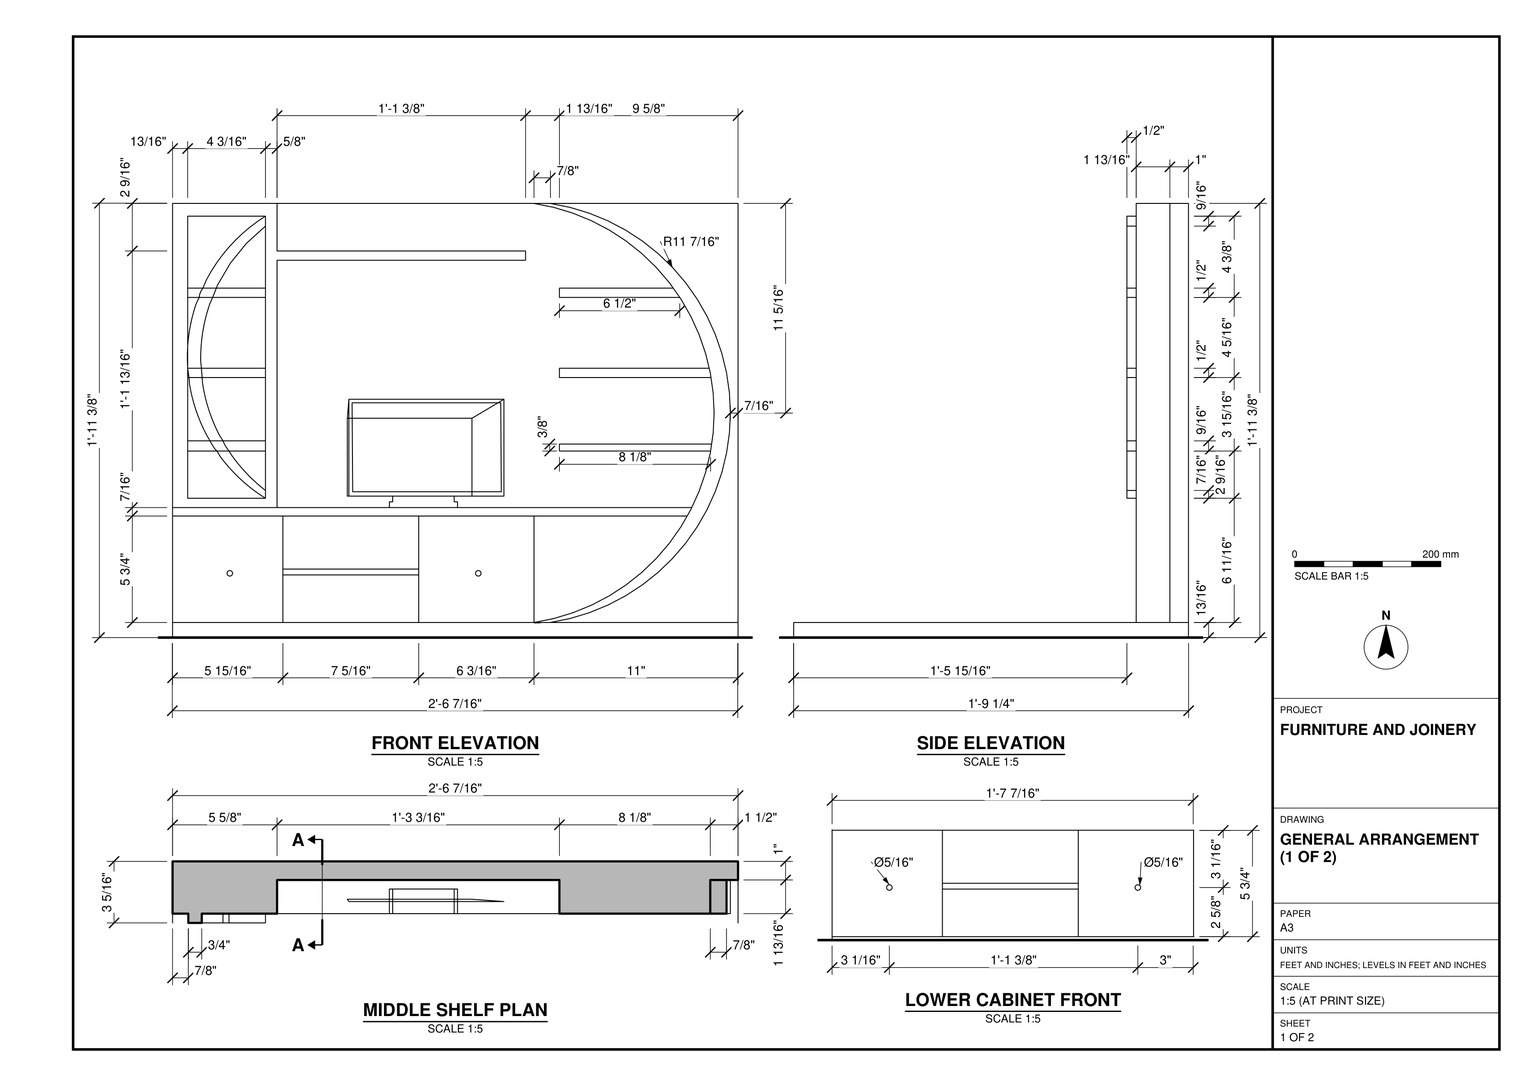
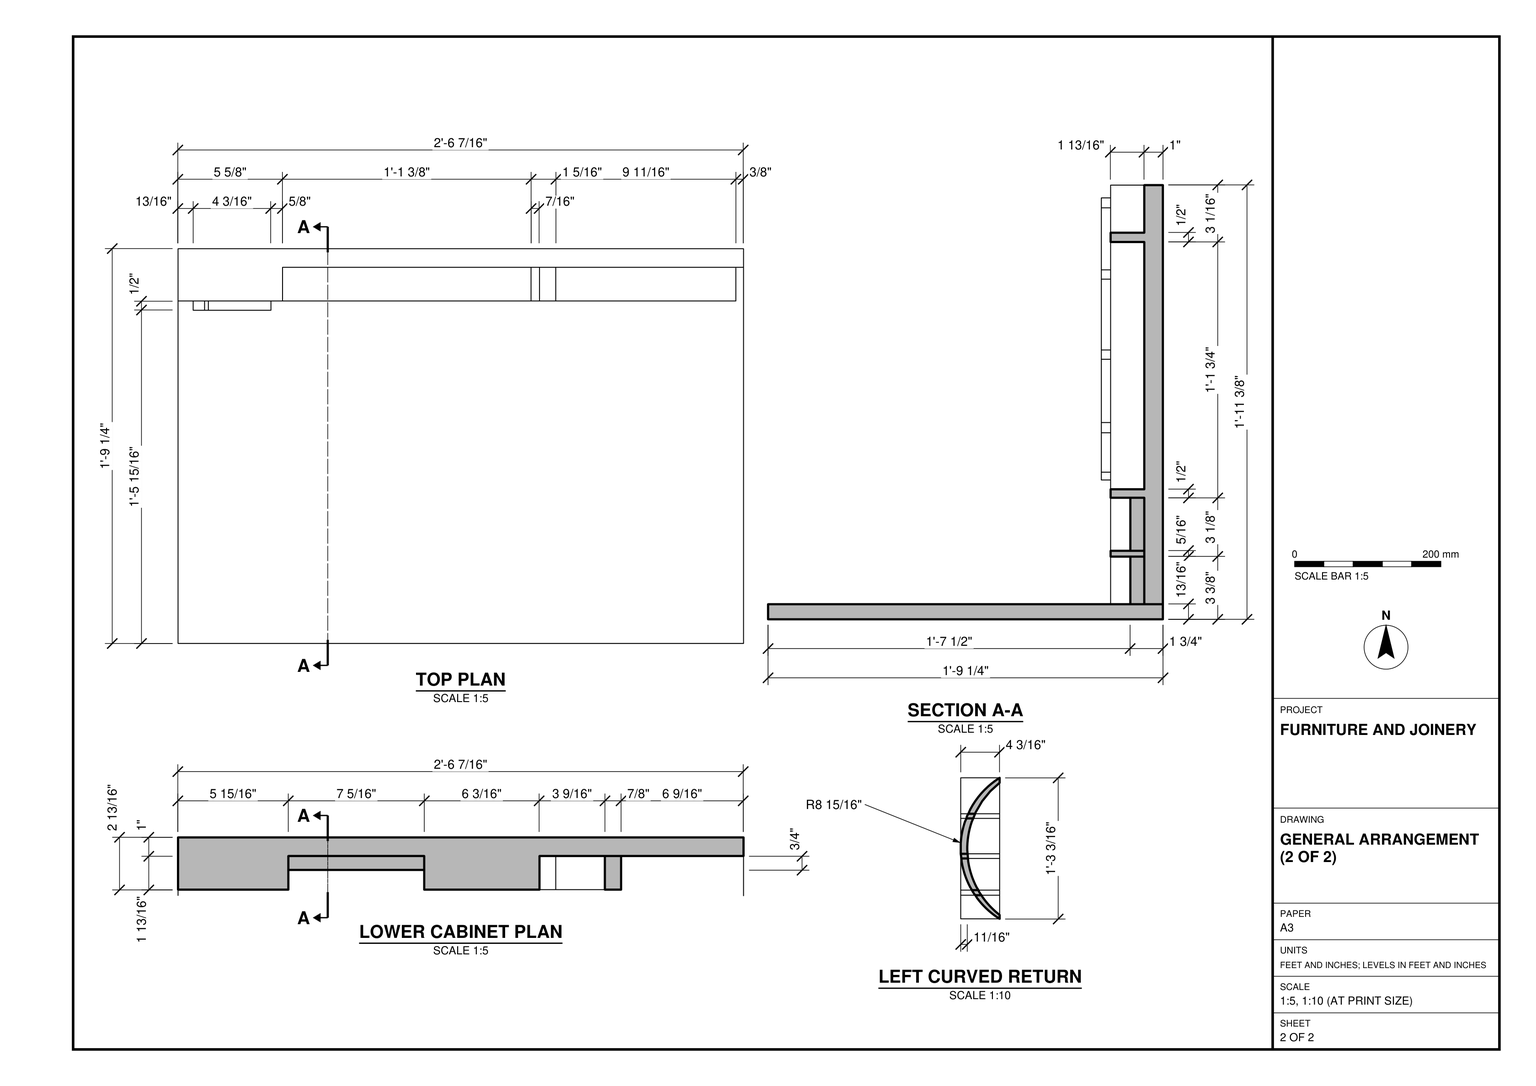
Use both sheets of task_files/diagram_01.pdf to model the television display unit in SketchUp. Work in feet and inches. Set the underside of the platform at ±0'-0". The complete unit is 2'-6 7/16" wide, 1'-9 1/4" deep and 1'-11 3/8" high. The depth includes the platform projecting in front of the shallow joinery; use the top plan and section to distinguish the platform footprint from the cabinet footprint.

Build the full-width platform and upright back panel. At the foot of the panel, place the lower cabinet with a knobbed front on either side of a recessed, shelved bay. Extend the display shelf above the cabinet to meet the large right-hand curve. Place the television on its stand in the central display space, with the short upper shelf extending into that space from the left. Use the curved-return detail for the narrow left shelving bay. On the right, follow the larger arc from the top of the unit down to the platform, fitting the three shelves to its inner edge.

Keep the platform, back panel, cabinet and other distinct joinery pieces in separate groups or components, and use components for repeated parts. Decor and loose items, including the television, may use any suitable library component. Save one SketchUp model as output_files/television_display_unit_with_curved_shelving.skp.

# SketchUp Ruby script. Lengths in inches.
U = 1.inch
M = Sketchup.active_model
def pt(a) = Geom::Point3d.new(a.map { |v| v * U })
def face(e, loops, mat)
  f = e.add_face(loops[0].map { |a| pt(a) })
  loops[1..].each { |l| e.add_face(l.map { |a| pt(a) }).erase! }
  f.material = f.back_material = mat if mat
  f
end
# faces: each face lists its corners as indices into pts; further lists are holes
def faces(e, pts, list, mat = nil) = list.each { |f| face(e, (f[0].is_a?(Array) ? f : [f]).map { |l| l.map { |i| pts[i] } }, mat) }
# xy, xz, yz: faces in a plane at the given z, y or x. An outline is a flat list of corners, or four numbers for a rectangle; further outlines are holes
def ring(l) = l.size == 4 ? [[l[0], l[1]], [l[2], l[1]], [l[2], l[3]], [l[0], l[3]]] : l.each_slice(2).to_a
def flat(e, list, mat, &to3) = list.each { |f| face(e, (f[0].is_a?(Array) ? f : [f]).map { |l| ring(l).map { |u, v| to3.(u, v) } }, mat) }
def xy(e, z, list, mat = nil) = flat(e, list, mat) { |x, y| [x, y, z] }
def xz(e, y, list, mat = nil) = flat(e, list, mat) { |x, z| [x, y, z] }
def yz(e, x, list, mat = nil) = flat(e, list, mat) { |y, z| [x, y, z] }
def lines(e, pts, list) = list.each { |a, b| e.add_line(pt(pts[a]), pt(pts[b])) }
# prism: a flat outline (further loops are holes) pulled along v
def prism(e, loops, v, mat = nil)
  f = face(e, loops, mat); d = Geom::Vector3d.new(v.map { |x| x * U })
  f.pushpull(f.normal.samedirection?(d) ? d.length : -d.length)
end
def box(e, o, s, mat = nil) = prism(e, [[o, [o[0] + s[0], o[1], o[2]], [o[0] + s[0], o[1] + s[1], o[2]], [o[0], o[1] + s[1], o[2]]]], [0, 0, s[2]], mat)
def at(x, y, z, deg = 0) = Geom::Transformation.translation(pt([x, y, z])) * Geom::Transformation.rotation(ORIGIN, Z_AXIS, deg.degrees)
def axes(o, x, y, z) = Geom::Transformation.new([*x, 0, *y, 0, *z, 0, *pt(o).to_a, 1])
def part(name) = M.definitions.add(name)
# library, detail: a bought-in or finely detailed component or shape, given as its bounding box
def library(name, o, s) = part(name).tap { |d| box(d.entities, o, s) }
def detail(e, o, s) = box(e.add_group.entities, o, s)
def put(e, d, t, mat = nil) = e.add_instance(d, t).tap { |i| i.material = mat if mat }
def group(e, t, mat = nil) = e.add_group.tap { |g| g.transformation = t; g.material = mat if mat }.entities
root = M.entities
M.materials.add("[0001_PaleVioletRed]").color = [219, 112, 147]
M.materials.add("[0005_LightPink]").color = [255, 182, 193]
M.materials.add("[0012_Bisque]").color = [255, 228, 196]
M.materials.add("[0131_Silver]").color = [192, 192, 192]
M.materials.add("[0132_LightGray]").color = [169, 169, 169]
M.materials.add("[0136_Charcoal]").color = [35, 35, 35]
M.materials.add("[Translucent Glass Gray]").color = [128, 128, 128]
M.materials["[Translucent Glass Gray]"].alpha = 0.5
M.materials.add("[Wood Bamboo]").color = [177, 105, 43]
M.materials.add("[Wood Floor Parquet]").color = [127, 78, 34]
xy(root,0,[[0,0,30.4375,21.25]])
xy(root,0.8125,[[0,18.4375,5.9375,20.25],[13.25,18.4375,13.25,20.25,0,20.25,0,21.25,30.4375,21.25,30.4375,20.25,17.19,20.25,17.19,18.4375],[17.19,18.4375,19.46,20.25],[19.46,18.4375,20.33,20.25],[5.9375,19.5,13.25,20.25]])
xy(root,0.8125,[[0,0,30.4375,0,30.4375,20.25,20.33,20.25,20.33,18.4375,13.25,18.4375,13.25,19.5,5.9375,19.5,5.9375,18.4375,0,18.4375]],"[0132_LightGray]")
xy(root,3.375,[[5.9375,18.4375,13.25,19.5],[5.9375,19.5,13.25,20.25]])
xy(root,3.6875,[[5.9375,19.5,13.25,20.25]])
xy(root,3.6875,[[5.9375,18.4375,13.25,19.5]],"[Wood Floor Parquet]")
xy(root,6.54,[[5.9375,19.5,13.25,20.25]])
xy(root,6.54,[[5.9375,18.4375,13.25,19.5],[19.46,18.4375,27.69,20.25]],"[Wood Bamboo]")
xy(root,7,[[5.625,18.4375,27.94,20.25]],"[Wood Floor Parquet]")
xy(root,7.5,[[0.8125,18.4375,5,20.25]],"[0005_LightPink]")
xy(root,10.04,[[2.38,17.9375,2.38,18.4375,0.8125,18.4375,0.8125,20.25,5,20.25,5,18.4375,3.04,18.4375,3.04,17.9375]])
xy(root,10.04,[[20.82,18.4375,28.96,20.25]],"[Wood Floor Parquet]")
xy(root,10.42,[[20.82,18.4375,29.01,20.25]],"[Wood Floor Parquet]")
xy(root,10.59,[[2.02,17.9375,2.71,17.9375,2.71,18.4375,5,18.4375,5,20.25,0.8125,20.25,0.8125,18.4375,2.02,18.4375]],"[Translucent Glass Gray]")
xy(root,14,[[0.89,17.9375,0.89,18.4375,0.8125,18.4375,0.8125,20.25,5,20.25,5,18.4375,1.59,18.4375,1.59,17.9375]],"[0005_LightPink]")
xy(root,14,[[20.82,18.4375,28.98,20.25]],"[Wood Floor Parquet]")
xy(root,14.5,[[0.8125,17.9375,1.55,17.9375,1.55,18.4375,5,18.4375,5,20.25,0.8125,20.25]],"[Translucent Glass Gray]")
xy(root,14.5,[[20.82,18.4375,28.88,20.25]],"[Wood Floor Parquet]")
xy(root,18.3125,[[1.43,17.9375,1.43,18.4375,0.8125,18.4375,0.8125,20.25,5,20.25,5,18.4375,2.16,18.4375,2.16,17.9375]],"[0005_LightPink]")
xy(root,18.3125,[[20.82,18.4375,27.3,20.25]],"[Wood Floor Parquet]")
xy(root,18.8125,[[1.63,17.9375,2.36,17.9375,2.36,18.4375,5,18.4375,5,20.25,0.8125,20.25,0.8125,18.4375,1.63,18.4375]],"[Translucent Glass Gray]")
xy(root,18.8125,[[20.82,18.4375,26.95,20.25]],"[Wood Floor Parquet]")
xy(root,20.3125,[[5.625,18.4375,19,20.25]],"[Wood Floor Parquet]")
xy(root,20.8125,[[5.625,18.4375,19,20.25]],"[Wood Floor Parquet]")
xy(root,22.6875,[[0.8125,18.4375,5,20.25]],"[0005_LightPink]")
xy(root,23.375,[[19.46,18.4375,20.33,20.25]],"[0001_PaleVioletRed]")
xy(root,23.375,[[0,18.4375,5.625,18.4375,5.625,20.25,30.4375,20.25,30.4375,21.25,0,21.25]],"[Wood Bamboo]")
xz(root,0,[[0,0,30.4375,0.8125]],"[0132_LightGray]")
xz(root,17.9375,[[5,7.5,5,7.92,4.77,8.1,4.55,8.29,4.34,8.49,4.13,8.6875,3.93,8.9,3.73,9.11,3.55,9.34,3.37,9.56,3.19,9.8,3.04,10.04,2.38,10.04,2.58,9.73,2.8,9.44,3.04,9.16,3.29,8.89,3.55,8.63,3.82,8.38,4.1,8.14,4.39,7.92,4.69,7.7],[2.38,10.04,3.04,10.04,2.91,10.22,2.8,10.4,2.71,10.59,2.02,10.59,2.09,10.45,2.27,10.17],[2.02,10.59,2.71,10.59,2.52,10.9,2.36,11.22,2.21,11.55,2.08,11.89,1.96,12.23,1.85,12.58,1.76,12.93,1.68,13.28,1.62,13.64,1.59,14,0.89,14,0.91,13.64,0.98,13.28,1.06,12.93,1.15,12.58,1.26,12.23,1.38,11.89,1.52,11.56,1.67,11.23,1.83,10.9],[0.89,14,1.59,14,1.55,14.5,0.8125,14.5],[0.8125,14.5,1.55,14.5,1.51,14.89,1.53,15.67,1.57,16.06,1.62,16.44,1.69,16.83,1.78,17.21,1.88,17.58,2,17.96,2.16,18.3125,1.43,18.3125,1.26,17.96,1.15,17.59,1.05,17.21,0.96,16.83,0.9,16.44,0.84,16.06,0.8125,15.68],
  [1.43,18.3125,2.16,18.3125,2.36,18.8125,1.63,18.8125,1.53,18.66,1.46,18.49],[1.63,18.8125,2.36,18.8125,2.43,18.99,3.12,20.17,3.99,21.23,5,22.15,5,22.6875,4.57,22.4,4.15,22.08,3.75,21.75,3.375,21.39,3.02,21,2.6875,20.6,2.38,20.18,2.09,19.74,1.84,19.29]],"[0001_PaleVioletRed]")
xz(root,18.4375,[[0.8125,14.5,0.8125,15.68,0.8125,15.67,0.79,15.28,0.8,14.89]])
xz(root,18.4375,[[19.46,0.8125,20.33,0.8125,21.39,1.03,22.42,1.34,23.42,1.75,24.38,2.25,25.28,2.84,26.13,3.51,26.91,4.26,27.61,5.07,28.23,5.96,28.77,6.89,29.22,7.875,29.57,8.9,29.82,9.95,29.97,11.02,30.02,12.09,29.97,13.17,29.82,14.24,29.57,15.29,29.22,16.3125,28.77,17.29,28.23,18.23,27.61,19.11,26.91,19.93,26.13,20.68,25.28,21.35,24.38,21.94,23.42,22.44,22.42,22.85,21.39,23.16,20.33,23.375,19.46,23.375,20.51,23.16,21.55,22.85,22.55,22.44,23.5,21.94,24.41,21.35,25.25,20.68,26.03,19.93,26.74,19.11,26.95,18.8125,27.3,18.3125,27.36,18.23,27.9,17.29,28.34,16.3125,28.69,15.29,28.88,14.5,28.95,14.24,28.98,14,29.1,13.17,29.15,12.09,29.1,11.02,29.01,10.42,28.96,10.04,28.95,9.95,28.69,8.9,28.34,7.875,27.94,7,27.9,6.89,27.69,6.54,27.36,5.96,26.74,5.07,26.03,4.26,25.25,3.51,24.41,2.84,23.5,2.25,22.55,1.75,21.55,1.34,20.51,1.03]],"[0001_PaleVioletRed]")
xz(root,18.4375,[[[0,0.8125,5.9375,6.54],[3.08,3.3125,3.04,3.32,3.01,3.33,2.98,3.35,2.95,3.38,2.9375,3.42,2.93,3.46,2.9375,3.5,2.95,3.53,2.97,3.57,3,3.59,3.04,3.61,3.12,3.61,3.15,3.59,3.1875,3.57,3.21,3.54,3.23,3.5,3.23,3.42,3.21,3.39,3.1875,3.36,3.16,3.33,3.12,3.32]],[[13.25,0.8125,19.46,6.54],[16.46,3.3125,16.42,3.32,16.38,3.33,16.35,3.35,16.33,3.38,16.3125,3.42,16.31,3.46,16.3125,3.5,16.33,3.53,16.35,3.57,16.38,3.59,16.42,3.61,16.49,3.61,16.53,3.59,16.5625,3.57,16.59,3.54,16.61,3.46,16.6,3.42,16.59,3.39,16.5625,3.36,16.53,3.33,16.5,3.32]]],"[0012_Bisque]")
xz(root,18.4375,[[3.08,3.3125,3.12,3.32,3.16,3.33,3.1875,3.36,3.21,3.39,3.23,3.42,3.23,3.5,3.21,3.54,3.1875,3.57,3.15,3.59,3.12,3.61,3.04,3.61,3,3.59,2.97,3.57,2.95,3.53,2.9375,3.5,2.93,3.46,2.9375,3.42,2.95,3.38,2.98,3.35,3.01,3.33,3.04,3.32],[16.46,3.3125,16.5,3.32,16.53,3.33,16.5625,3.36,16.59,3.39,16.6,3.42,16.61,3.46,16.59,3.54,16.5625,3.57,16.53,3.59,16.49,3.61,16.42,3.61,16.38,3.59,16.35,3.57,16.33,3.53,16.3125,3.5,16.31,3.46,16.3125,3.42,16.33,3.38,16.35,3.35,16.38,3.33,16.42,3.32]],"[0132_LightGray]")
xz(root,18.4375,[[0.8125,10.04,2.38,10.04,2.27,10.17,2.09,10.45,2.02,10.59,0.8125,10.59],[3.04,10.04,5,10.04,5,10.59,2.71,10.59,2.8,10.4,2.91,10.22],[1.59,14,5,14,5,14.5,1.55,14.5],[0.8125,18.3125,1.43,18.3125,1.46,18.49,1.53,18.66,1.63,18.8125,0.8125,18.8125],[2.16,18.3125,5,18.3125,5,18.8125,2.36,18.8125]],"[Translucent Glass Gray]")
xz(root,18.4375,[[5.9375,3.375,13.25,3.6875],[0,6.54,27.69,6.54,27.9,6.89,27.94,7,0,7],[[0,7,5.625,7,5.625,20.3125,19,20.3125,19,20.8125,5.625,20.8125,5.625,23.375,0,23.375],[0.8125,7.5,0.8125,14.5,0.8,14.89,0.79,15.28,0.8125,15.67,0.8125,22.6875,5,22.6875,5,7.5]],[20.82,10.04,28.96,10.04,29.01,10.42,20.82,10.42],[0.8125,14,0.89,14,0.8125,14.5],
  [20.82,14,28.98,14,28.95,14.24,28.88,14.5,20.82,14.5],[20.82,18.3125,27.3,18.3125,26.95,18.8125,20.82,18.8125]],"[Wood Floor Parquet]")
xz(root,19.5,[[5.9375,0.8125,13.25,3.375],[5.9375,3.6875,13.25,6.54]],"[Wood Floor Parquet]")
xz(root,20.25,[[17.56,0.73,20.33,0.8125,17.19,0.8125],[5.9375,0.8125,13.25,3.375],[19.46,0.8125,20.51,1.03,21.55,1.34,22.55,1.75,23.5,2.25,24.41,2.84,25.09,3.375,25.25,3.51,25.44,3.6875,26.03,4.26,26.74,5.07,27.36,5.96,27.69,6.54,27.9,6.89,27.94,7,28.34,7.875,28.69,8.9,28.95,9.95,28.96,10.04,29.01,10.42,29.1,11.02,29.15,12.09,29.1,13.17,28.98,14,28.95,14.24,28.88,14.5,28.69,15.29,28.34,16.3125,27.9,17.29,27.36,18.23,27.3,18.3125,26.95,18.8125,26.74,19.11,26.03,19.93,25.25,20.68,24.41,21.35,23.5,21.94,22.55,22.44,21.55,22.85,20.51,23.16,19.46,23.375,20.33,23.375,21.39,23.16,22.42,22.85,23.42,22.44,24.38,21.94,25.28,21.35,26.13,20.68,26.91,19.93,27.61,19.11,28.23,18.23,28.77,17.29,29.22,16.3125,29.57,15.29,29.82,14.24,29.97,13.17,30.02,12.09,29.97,11.02,29.82,9.95,29.57,8.9,29.22,7.875,28.77,6.89,28.23,5.96,27.61,5.07,26.91,4.26,26.13,3.51,25.28,2.84,24.38,2.25,23.42,1.75,22.42,1.34,21.39,1.03,20.33,0.8125],[5.9375,3.375,13.25,3.6875],[5.9375,3.6875,13.25,6.54]])
xz(root,20.25,[[0.8125,7.5,5,10.04],[0.8125,10.59,5,14],[0.8125,14.5,5,18.3125],[0.8125,18.8125,5,22.6875]],"[0005_LightPink]")
xz(root,20.25,[[19.46,0.8125,20.51,1.03,21.55,1.34,22.55,1.75,23.5,2.25,24.41,2.84,25.09,3.375,25.25,3.51,25.44,3.6875,26.03,4.26,26.74,5.07,27.36,5.96,27.69,6.54,19.46,6.54],[20.33,0.8125,30.4375,0.8125,30.4375,23.375,20.33,23.375,21.39,23.16,22.42,22.85,23.42,22.44,24.38,21.94,25.28,21.35,26.13,20.68,26.91,19.93,27.61,19.11,28.23,18.23,28.77,17.29,29.22,16.3125,29.57,15.29,29.82,14.24,29.97,13.17,30.02,12.09,29.97,11.02,29.82,9.95,29.57,8.9,29.22,7.875,28.77,6.89,28.23,5.96,27.61,5.07,26.91,4.26,26.13,3.51,25.28,2.84,24.38,2.25,23.42,1.75,22.42,1.34,21.39,1.03],[5.625,7,27.94,7,28.34,7.875,28.69,8.9,28.95,9.95,28.96,10.04,20.82,10.04,20.82,10.42,29.01,10.42,29.1,11.02,29.15,12.09,29.1,13.17,28.98,14,20.82,14,20.82,14.5,28.88,14.5,28.69,15.29,28.34,16.3125,27.9,17.29,27.36,18.23,27.3,18.3125,20.82,18.3125,20.82,18.8125,26.95,18.8125,26.74,19.11,26.03,19.93,25.25,20.68,24.41,21.35,23.5,21.94,22.55,22.44,21.55,22.85,20.51,23.16,19.46,23.375,5.625,23.375,5.625,20.8125,19,20.8125,19,20.3125,5.625,20.3125]],"[0012_Bisque]")
xz(root,21.25,[[0,0,30.4375,0.8125],[0,0.8125,30.4375,23.375]],"[0132_LightGray]")
yz(root,0,[[18.4375,0.8125,21.25,6.54]],"[0012_Bisque]")
yz(root,0,[[0,0,21.25,0.8125]],"[0132_LightGray]")
yz(root,0,[[18.4375,6.54,21.25,23.375]],"[Wood Bamboo]")
yz(root,0.8125,[[17.9375,14.5,18.4375,15.68]],"[0001_PaleVioletRed]")
yz(root,0.8125,[[18.4375,7.5,20.25,10.04],[18.4375,10.59,20.25,14],[18.4375,14.5,20.25,18.3125],[18.4375,18.8125,20.25,22.6875]],"[0005_LightPink]")
yz(root,5,[[17.9375,7.5,18.4375,7.92],[17.9375,22.15,18.4375,22.6875]],"[0001_PaleVioletRed]")
yz(root,5,[[18.4375,7.5,20.25,10.04],[18.4375,10.59,20.25,14],[18.4375,14.5,20.25,18.3125],[18.4375,18.8125,20.25,22.6875]],"[0005_LightPink]")
yz(root,5.625,[[18.4375,20.8125,20.25,23.375]],"[Wood Bamboo]")
yz(root,5.625,[[18.4375,7,20.25,20.3125]],"[Wood Floor Parquet]")
yz(root,5.9375,[[19.5,0.8125,20.25,3.375],[18.4375,3.375,20.25,3.6875],[19.5,3.6875,20.25,6.54]])
yz(root,5.9375,[[18.4375,0.8125,19.5,3.375],[18.4375,3.6875,19.5,6.54]],"[Wood Floor Parquet]")
yz(root,13.25,[[19.5,0.8125,20.25,3.375],[18.4375,3.375,20.25,3.6875],[19.5,3.6875,20.25,6.54]])
yz(root,13.25,[[18.4375,0.8125,19.5,3.375],[18.4375,3.6875,19.5,6.54]],"[Wood Bamboo]")
yz(root,19,[[18.4375,20.3125,20.25,20.8125]],"[Wood Floor Parquet]")
yz(root,19.46,[[18.4375,0.8125,20.25,6.54]],"[0012_Bisque]")
yz(root,20.82,[[18.4375,10.04,20.25,10.42],[18.4375,14,20.25,14.5],[18.4375,18.3125,20.25,18.8125]],"[Wood Floor Parquet]")
yz(root,30.4375,[[20.25,0.8125,21.25,23.375]],"[0012_Bisque]")
yz(root,30.4375,[[0,0,21.25,0.8125]],"[0132_LightGray]")
p = [[20.51,20.25,1.03],[19.46,20.25,0.8125],[19.46,18.4375,0.8125],[20.51,18.4375,1.03],[20.33,20.25,0.8125],[21.39,20.25,1.03],
  [21.39,18.4375,1.03],[20.33,18.4375,0.8125],[21.55,20.25,1.34],[21.55,18.4375,1.34],[22.42,20.25,1.34],[22.42,18.4375,1.34],
  [22.55,20.25,1.75],[22.55,18.4375,1.75],[23.42,20.25,1.75],[23.42,18.4375,1.75],[23.5,20.25,2.25],[23.5,18.4375,2.25],
  [24.38,20.25,2.25],[24.38,18.4375,2.25],[24.41,20.25,2.84],[24.41,18.4375,2.84],[25.28,20.25,2.84],[25.28,18.4375,2.84],
  [25.25,20.25,3.51],[25.09,20.25,3.375],[25.25,18.4375,3.51],[26.13,20.25,3.51],[26.13,18.4375,3.51],[26.03,20.25,4.26],
  [25.44,20.25,3.6875],[26.03,18.4375,4.26],[26.91,20.25,4.26],[26.91,18.4375,4.26],[26.74,20.25,5.07],[26.74,18.4375,5.07],
  [27.61,20.25,5.07],[27.61,18.4375,5.07],[27.36,20.25,5.96],[27.36,18.4375,5.96],[28.23,20.25,5.96],[28.23,18.4375,5.96],
  [27.69,18.4375,6.54],[27.69,20.25,6.54],[28.77,20.25,6.89],[28.77,18.4375,6.89],[27.9,20.25,6.89],[27.9,18.4375,6.89],
  [27.94,18.4375,7],[27.94,20.25,7],[29.22,20.25,7.875],[29.22,18.4375,7.875],[28.34,20.25,7.875],[28.34,18.4375,7.875],
  [4.69,18.4375,7.7],[5,18.4375,7.5],[5,17.9375,7.5],[4.69,17.9375,7.7],[4.39,18.4375,7.92],[4.39,17.9375,7.92],
  [4.1,18.4375,8.14],[4.1,17.9375,8.14],[5,18.4375,7.92],[4.77,18.4375,8.1],[4.77,17.9375,8.1],[5,17.9375,7.92],
  [28.69,20.25,8.9],[28.69,18.4375,8.9],[29.57,20.25,8.9],[29.57,18.4375,8.9],[3.82,18.4375,8.38],[3.82,17.9375,8.38],
  [4.55,18.4375,8.29],[4.55,17.9375,8.29],[4.34,18.4375,8.49],[4.34,17.9375,8.49],[3.55,18.4375,8.63],[3.55,17.9375,8.63],
  [4.13,18.4375,8.6875],[4.13,17.9375,8.6875],[3.29,18.4375,8.89],[3.29,17.9375,8.89],[3.93,18.4375,8.9],[3.93,17.9375,8.9],
  [3.04,18.4375,9.16],[3.04,17.9375,9.16],[3.73,18.4375,9.11],[3.73,17.9375,9.11],[28.95,20.25,9.95],[28.95,18.4375,9.95],
  [29.82,20.25,9.95],[29.82,18.4375,9.95],[3.55,18.4375,9.34],[3.55,17.9375,9.34],[2.8,18.4375,9.44],[2.8,17.9375,9.44],
  [3.37,18.4375,9.56],[3.37,17.9375,9.56],[2.58,18.4375,9.73],[2.58,17.9375,9.73],[3.19,18.4375,9.8],[3.19,17.9375,9.8],
  [2.38,18.4375,10.04],[2.38,17.9375,10.04],[3.04,18.4375,10.04],[3.04,17.9375,10.04],[28.96,18.4375,10.04],[28.96,20.25,10.04],
  [29.97,20.25,11.02],[29.97,18.4375,11.02],[2.27,18.4375,10.17],[2.27,17.9375,10.17],[2.91,18.4375,10.22],[2.91,17.9375,10.22],
  [29.01,20.25,10.42],[29.01,18.4375,10.42],[2.18,18.4375,10.31],[2.18,17.9375,10.31],[2.8,18.4375,10.4],[2.8,17.9375,10.4],
  [2.09,18.4375,10.45],[2.09,17.9375,10.45],[2.02,18.4375,10.59],[2.02,17.9375,10.59],[2.71,18.4375,10.59],[2.71,17.9375,10.59],
  [29.1,20.25,11.02],[29.1,18.4375,11.02],[1.83,18.4375,10.9],[1.83,17.9375,10.9],[2.52,18.4375,10.9],[2.52,17.9375,10.9],
  [1.67,18.4375,11.23],[1.67,17.9375,11.23],[2.36,18.4375,11.22],[2.36,17.9375,11.22],[29.15,20.25,12.09],[29.15,18.4375,12.09],
  [30.02,20.25,12.09],[30.02,18.4375,12.09],[1.52,18.4375,11.56],[1.52,17.9375,11.56],[2.21,18.4375,11.55],[2.21,17.9375,11.55],
  [1.38,18.4375,11.89],[1.38,17.9375,11.89],[2.08,18.4375,11.89],[2.08,17.9375,11.89],[1.26,18.4375,12.23],[1.26,17.9375,12.23],
  [1.96,18.4375,12.23],[1.96,17.9375,12.23],[29.1,20.25,13.17],[29.1,18.4375,13.17],[29.97,20.25,13.17],[29.97,18.4375,13.17],
  [1.15,18.4375,12.58],[1.15,17.9375,12.58],[1.85,18.4375,12.58],[1.85,17.9375,12.58],[1.06,18.4375,12.93],[1.06,17.9375,12.93],
  [1.76,18.4375,12.93],[1.76,17.9375,12.93],[0.98,18.4375,13.28],[0.98,17.9375,13.28],[1.68,18.4375,13.28],[1.68,17.9375,13.28],
  [28.98,18.4375,14],[28.98,20.25,14],[29.82,20.25,14.24],[29.82,18.4375,14.24],[0.91,18.4375,13.64],[0.91,17.9375,13.64],
  [1.62,18.4375,13.64],[1.62,17.9375,13.64],[0.89,18.4375,14],[0.89,17.9375,14],[1.59,18.4375,14],[1.59,17.9375,14],
  [0.8125,18.4375,14.5],[0.8125,17.9375,14.5],[1.55,18.4375,14.5],[1.55,17.9375,14.5],[28.95,20.25,14.24],[28.95,18.4375,14.24],
  [28.88,20.25,14.5],[28.88,18.4375,14.5],[29.57,20.25,15.29],[29.57,18.4375,15.29],[1.51,18.4375,14.89],[1.51,17.9375,14.89],
  [28.69,20.25,15.29],[28.69,18.4375,15.29],[1.52,18.4375,15.28],[1.52,17.9375,15.28],[1.53,18.4375,15.67],[1.53,17.9375,15.67],
  [28.34,20.25,16.3125],[28.34,18.4375,16.3125],[29.22,20.25,16.3125],[29.22,18.4375,16.3125],[0.84,18.4375,16.06],[0.8125,18.4375,15.68],
  [0.8125,17.9375,15.68],[0.84,17.9375,16.06],[1.57,18.4375,16.06],[1.57,17.9375,16.06],[0.9,18.4375,16.44],[0.9,17.9375,16.44],
  [1.62,18.4375,16.44],[1.62,17.9375,16.44],[27.9,20.25,17.29],[27.9,18.4375,17.29],[28.77,20.25,17.29],[28.77,18.4375,17.29],
  [0.96,18.4375,16.83],[0.96,17.9375,16.83],[1.69,18.4375,16.83],[1.69,17.9375,16.83],[1.05,18.4375,17.21],[1.05,17.9375,17.21],
  [1.78,18.4375,17.21],[1.78,17.9375,17.21],[1.15,18.4375,17.59],[1.15,17.9375,17.59],[1.88,18.4375,17.58],[1.88,17.9375,17.58],
  [27.36,20.25,18.23],[27.36,18.4375,18.23],[28.23,20.25,18.23],[28.23,18.4375,18.23],[1.26,18.4375,17.96],[1.26,17.9375,17.96],
  [2,18.4375,17.96],[2,17.9375,17.96],[1.43,18.4375,18.3125],[1.43,17.9375,18.3125],[2.16,18.4375,18.3125],[2.16,17.9375,18.3125],
  [27.3,18.4375,18.3125],[27.3,20.25,18.3125],[27.61,20.25,19.11],[27.61,18.4375,19.11],[1.46,18.4375,18.49],[1.46,17.9375,18.49],
  [2.36,18.4375,18.8125],[2.36,17.9375,18.8125],[26.95,20.25,18.8125],[26.95,18.4375,18.8125],[1.53,18.4375,18.66],[1.53,17.9375,18.66],
  [1.63,18.4375,18.8125],[1.63,17.9375,18.8125],[1.84,18.4375,19.29],[1.84,17.9375,19.29],[2.43,18.4375,18.99],[2.43,17.9375,18.99],
  [26.74,20.25,19.11],[26.74,18.4375,19.11],[3.12,18.4375,20.17],[3.12,17.9375,20.17],[26.03,20.25,19.93],[26.03,18.4375,19.93],
  [26.91,20.25,19.93],[26.91,18.4375,19.93],[2.09,18.4375,19.74],[2.09,17.9375,19.74],[2.38,18.4375,20.18],[2.38,17.9375,20.18],
  [25.25,20.25,20.68],[25.25,18.4375,20.68],[26.13,20.25,20.68],[26.13,18.4375,20.68],[2.6875,18.4375,20.6],[2.6875,17.9375,20.6],
  [3.99,18.4375,21.23],[3.99,17.9375,21.23],[3.02,18.4375,21],[3.02,17.9375,21],[24.41,20.25,21.35],[24.41,18.4375,21.35],
  [25.28,20.25,21.35],[25.28,18.4375,21.35],[3.375,18.4375,21.39],[3.375,17.9375,21.39],[5,18.4375,22.15],[5,17.9375,22.15],
  [3.75,18.4375,21.75],[3.75,17.9375,21.75],[23.5,20.25,21.94],[23.5,18.4375,21.94],[24.38,20.25,21.94],[24.38,18.4375,21.94],
  [4.15,18.4375,22.08],[4.15,17.9375,22.08],[22.55,20.25,22.44],[22.55,18.4375,22.44],[23.42,20.25,22.44],[23.42,18.4375,22.44],
  [4.57,18.4375,22.4],[4.57,17.9375,22.4],[5,18.4375,22.6875],[5,17.9375,22.6875],[21.55,20.25,22.85],[21.55,18.4375,22.85],
  [22.42,20.25,22.85],[22.42,18.4375,22.85],[20.51,20.25,23.16],[20.51,18.4375,23.16],[21.39,20.25,23.16],[21.39,18.4375,23.16],
  [19.46,20.25,23.375],[19.46,18.4375,23.375],[20.33,20.25,23.375],[20.33,18.4375,23.375]]
faces(root,p,[[0,1,2,3],[4,5,6,7],[8,0,3,9],[5,10,11,6],[12,8,9,13],[10,14,15,11],[16,12,13,17],[14,18,19,15],
  [20,16,17,21],[18,22,23,19],[24,25,20,21,26],[22,27,28,23],[29,30,24,26,31],[27,32,33,28],[34,29,31,35],[32,36,37,33],
  [38,34,35,39],[36,40,41,37],[39,42,43,38],[40,44,45,41],[44,50,51,45],[52,49,48,53],[54,55,56,57],[58,54,57,59],
  [60,58,59,61],[62,63,64,65],[66,52,53,67],[50,68,69,51],[70,60,61,71],[63,72,73,64],[72,74,75,73],[76,70,71,77],
  [74,78,79,75],[80,76,77,81],[78,82,83,79],[84,80,81,85],[82,86,87,83],[88,66,67,89],[68,90,91,69],[86,92,93,87],
  [94,84,85,95],[92,96,97,93],[98,94,95,99],[96,100,101,97],[102,98,99,103],[100,104,105,101],[89,106,107,88],[90,108,109,91],
  [110,102,103,111],[104,112,113,105],[116,110,111,117],[112,118,119,113],[120,116,117,121],[122,120,121,123],[118,124,125,119],[126,114,115,127],
  [128,122,123,129],[124,130,131,125],[132,128,129,133],[130,134,135,131],[136,126,127,137],[108,138,139,109],[140,132,133,141],[134,142,143,135],
  [144,140,141,145],[142,146,147,143],[148,144,145,149],[146,150,151,147],[152,136,137,153],[138,154,155,139],[156,148,149,157],[150,158,159,151],
  [160,156,157,161],[158,162,163,159],[164,160,161,165],[162,166,167,163],[153,168,169,152],[154,170,171,155],[172,164,165,173],[166,174,175,167],
  [176,172,173,177],[174,178,179,175],[180,176,177,181],[178,182,183,179],[170,188,189,171],[182,190,191,183],[192,186,187,193],[190,194,195,191],
  [194,196,197,195],[198,192,193,199],[188,200,201,189],[202,203,204,205],[196,206,207,197],[208,202,205,209],[206,210,211,207],[212,198,199,213],
  [200,214,215,201],[216,208,209,217],[210,218,219,211],[220,216,217,221],[218,222,223,219],[224,220,221,225],[222,226,227,223],[228,212,213,229],
  [214,230,231,215],[232,224,225,233],[226,234,235,227],[236,232,233,237],[234,238,239,235],[229,240,241,228],[230,242,243,231],[244,236,237,245],
  [238,246,247,239],[250,244,245,251],[252,250,251,253],[254,252,253,255],[246,256,257,247],[258,248,249,259],[256,260,261,257],[262,258,259,263],
  [242,264,265,243],[266,254,255,267],[268,266,267,269],[270,262,263,271],[264,272,273,265],[274,268,269,275],[260,276,277,261],[278,274,275,279],
  [280,270,271,281],[272,282,283,273],[284,278,279,285],[276,286,287,277],[288,284,285,289],[290,280,281,291],[282,292,293,283],[294,288,289,295],
  [296,290,291,297],[292,298,299,293],[300,294,295,301],[302,300,301,303],[304,296,297,305],[298,306,307,299],[308,304,305,309],[306,310,311,307],
  [312,308,309,313],[310,314,315,311]],"[0001_PaleVioletRed]")
faces(root,p,[[46,43,42,47],[47,48,49,46],[114,107,106,115],[184,169,168,185],[186,184,185,187],[248,241,240,249]])
g1 = group(root,at(11.67,18.4375,7),"[0136_Charcoal]")
prism(g1,[[[0,0,0],[3.67,0,0],[3.67,0,0.31],[3.49,0,0.31],[3.49,0,0.62],[0.18,0,0.62],[0.18,0,0.31],[0,0,0.31]]],[0,1.32,0])
g2 = group(root,at(9.41,19.09,7.62),"[0131_Silver]")
xy(g2,0,[[0.08,0,0,0.125,6.71,0.125,8.43,0]])
xz(g2,0,[[0.29,0.24,8.29,0.24,8.26,5.02,0.26,5.02]])
xz(g2,0,[[[0.08,0,8.43,5.21],[0.29,0.24,0.26,5.02,8.26,5.02,8.29,0.24]]],"[0136_Charcoal]")
xz(g2,0.125,[[0,0,6.71,4.19]])
p = [[0.08,0,5.21],[0,0.125,4.19],[0,0.125,0],[0.08,0,0],[6.71,0.125,0],[6.71,0.125,4.19],
  [8.43,0,5.21],[8.43,0,0]]
faces(g2,p,[[0,1,2,3],[4,5,6,7],[1,0,6,5]])
